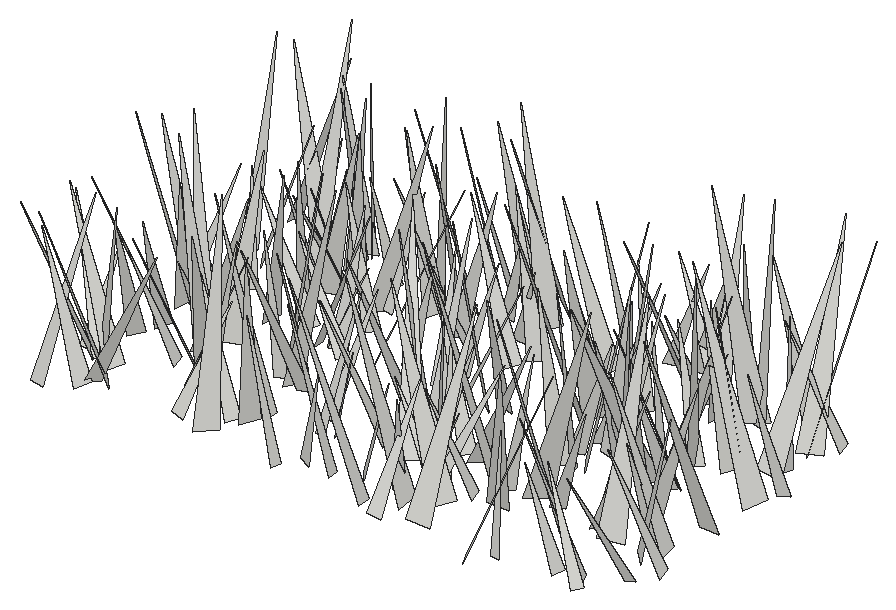
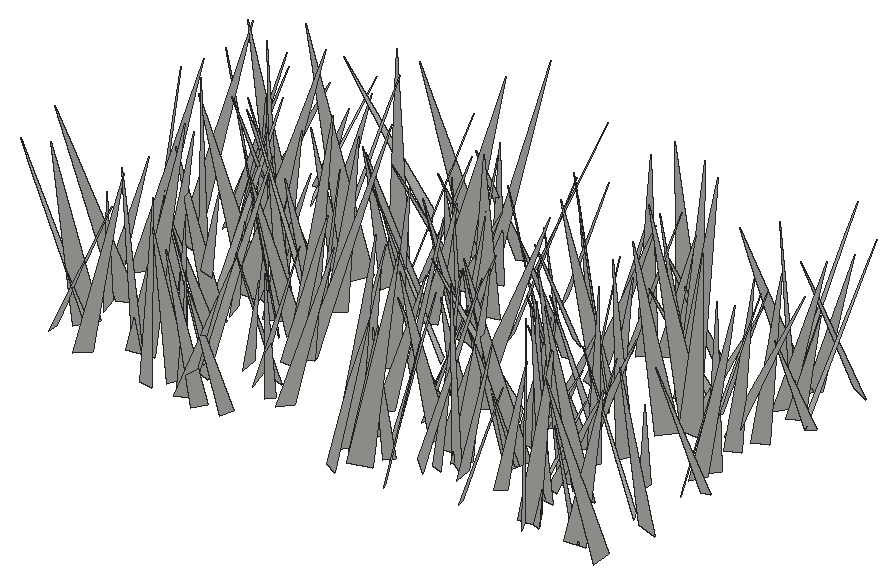
# SketchUp Ruby script. Lengths in inches.
U = 1.inch
M = Sketchup.active_model
def pt(a) = Geom::Point3d.new(a.map { |v| v * U })
def face(e, loops, mat)
  f = e.add_face(loops[0].map { |a| pt(a) })
  loops[1..].each { |l| e.add_face(l.map { |a| pt(a) }).erase! }
  f.material = f.back_material = mat if mat
  f
end
# faces: each face lists its corners as indices into pts; further lists are holes
def faces(e, pts, list, mat = nil) = list.each { |f| face(e, (f[0].is_a?(Array) ? f : [f]).map { |l| l.map { |i| pts[i] } }, mat) }
# xy, xz, yz: faces in a plane at the given z, y or x. An outline is a flat list of corners, or four numbers for a rectangle; further outlines are holes
def ring(l) = l.size == 4 ? [[l[0], l[1]], [l[2], l[1]], [l[2], l[3]], [l[0], l[3]]] : l.each_slice(2).to_a
def flat(e, list, mat, &to3) = list.each { |f| face(e, (f[0].is_a?(Array) ? f : [f]).map { |l| ring(l).map { |u, v| to3.(u, v) } }, mat) }
def xy(e, z, list, mat = nil) = flat(e, list, mat) { |x, y| [x, y, z] }
def xz(e, y, list, mat = nil) = flat(e, list, mat) { |x, z| [x, y, z] }
def yz(e, x, list, mat = nil) = flat(e, list, mat) { |y, z| [x, y, z] }
def lines(e, pts, list) = list.each { |a, b| e.add_line(pt(pts[a]), pt(pts[b])) }
# prism: a flat outline (further loops are holes) pulled along v
def prism(e, loops, v, mat = nil)
  f = face(e, loops, mat); d = Geom::Vector3d.new(v.map { |x| x * U })
  f.pushpull(f.normal.samedirection?(d) ? d.length : -d.length)
end
def box(e, o, s, mat = nil) = prism(e, [[o, [o[0] + s[0], o[1], o[2]], [o[0] + s[0], o[1] + s[1], o[2]], [o[0], o[1] + s[1], o[2]]]], [0, 0, s[2]], mat)
def at(x, y, z, deg = 0) = Geom::Transformation.translation(pt([x, y, z])) * Geom::Transformation.rotation(ORIGIN, Z_AXIS, deg.degrees)
def axes(o, x, y, z) = Geom::Transformation.new([*x, 0, *y, 0, *z, 0, *pt(o).to_a, 1])
def part(name) = M.definitions.add(name)
# library, detail: a bought-in or finely detailed component or shape, given as its bounding box
def library(name, o, s) = part(name).tap { |d| box(d.entities, o, s) }
def detail(e, o, s) = box(e.add_group.entities, o, s)
def put(e, d, t, mat = nil) = e.add_instance(d, t).tap { |i| i.material = mat if mat }
def group(e, t, mat = nil) = e.add_group.tap { |g| g.transformation = t; g.material = mat if mat }.entities
root = M.entities
c1 = part("fur_instance\#9")
p = [[0.8125,0,1.79],[0.67,-0.02,1.48],[0,-0.11,0],[0,0.11,0]]
faces(c1.entities,p,[[0,1,2,3]])
put(root,c1,axes([494.55,409.32,-21.66],[-3.60372,1.36671,1.25031],[1.68423,3.55609,0.96723],[0.77106,-1.37995,3.73084]))
put(root,c1,axes([458.37,410.72,-21.66],[-4.85913,-4.7221,0.69622],[-4.68141,4.90862,0.61965],[0.93132,0.03646,6.74725]))
put(root,c1,axes([496.72,408.43,-21.66],[-1.92431,3.57441,0.40694],[3.46774,1.72017,1.28872],[-0.95749,-0.95373,3.84949]))
put(root,c1,axes([479.86,408.75,-21.66],[-7.1325,-1.97369,0.04131],[-1.9512,7.0246,-1.27181],[-0.29997,1.23662,7.29044]))
put(root,c1,axes([457.51,409.38,-21.66],[-4.78062,2.36193,1.12593],[2.54726,4.73726,0.87783],[0.59826,-1.2963,5.25951]))
put(root,c1,axes([490.34,408.35,-21.66],[1.055,3.81063,1.04337],[3.83467,-1.24762,0.6792],[-0.95124,-0.80317,3.89521]))
put(root,c1,axes([489.08,407.03,-21.66],[5.73522,3.47371,0.17785],[3.39582,-5.66618,1.16354],[-0.75282,0.90483,6.60345]))
put(root,c1,axes([481.44,407.72,-21.66],[-0.33332,4.6985,0.41104],[4.65173,0.39553,-0.74898],[0.77866,-0.35159,4.65038]))
put(root,c1,axes([496.18,409.8,-21.66],[-4.80301,-2.64529,0.12183],[-2.62964,4.73476,-0.865],[-0.31202,0.81591,5.41463]))
put(root,c1,axes([481.99,410.3,-21.66],[-7.83608,-0.63477,1.59162],[-0.4911,7.96997,0.76075],[1.64165,-0.64574,7.82485]))
put(root,c1,axes([472.91,408.91,-21.66],[-4.76571,-0.2474,0.30777],[-0.30187,4.68534,-0.90794],[0.25457,0.92426,4.68496]))
put(root,c1,axes([498.58,411.23,-21.66],[-0.19761,-4.29399,0.26182],[-4.09062,0.10641,-1.34218],[-1.33181,0.31028,4.08362]))
put(root,c1,axes([480.77,411.1,-21.66],[0.8236,-4.35079,0.44599],[-4.32851,-0.74586,0.71716],[0.62636,0.56649,4.3696]))
put(root,c1,axes([473.95,410.375,-21.66],[-0.58036,-3.55618,1.37675],[-3.59236,0.97706,1.00942],[1.27936,1.13031,3.45894]))
put(root,c1,axes([457.67,410.2,-21.66],[5.28703,-2.12696,0.17156],[-2.11759,-5.17319,1.12251],[0.26309,1.10465,5.58719]))
put(root,c1,axes([455.2,407.84,-21.66],[2.05142,5.93925,0.09208],[5.90467,-2.04959,0.65232],[-0.64654,0.12643,6.2496]))
put(root,c1,axes([484.12,408.71,-21.66],[-1.25446,7.26591,1.58891],[7.27727,1.53186,-1.25954],[1.53602,-1.32352,7.26503]))
put(root,c1,axes([476.24,410.25,-21.66],[-5.31837,-1.43549,0.4315],[-1.49067,5.23198,-0.96754],[0.15722,1.04767,5.42306]))
put(root,c1,axes([483.2,409.68,-21.66],[3.56009,0.21869,0.65734],[0.01468,-3.46445,1.07311],[-0.69261,1.05069,3.40155]))
put(root,c1,axes([455.43,412.93,-21.66],[-4.61159,-4.4726,0.38091],[-4.39573,4.61032,0.9157],[0.90928,-0.396,6.35865]))
put(root,c1,axes([466.86,409.73,-21.66],[-5.99811,4.4385,2.51735],[4.45899,6.44808,-0.74453],[2.48087,-0.8583,7.4245]))
put(root,c1,axes([468.24,412.22,-21.66],[5.51508,-3.1001,1.56666],[-3.03836,-5.73026,-0.64316],[-1.68328,0.18611,6.29389]))
put(root,c1,axes([477.88,411.24,-21.66],[3.15545,2.01724,0.79775],[2.15051,-3.09372,-0.68323],[-0.2846,-1.01105,3.6823]))
put(root,c1,axes([464.3,410.09,-21.66],[0.4921,4.23207,0.57816],[4.10963,-0.31046,-1.22532],[1.16432,-0.69285,4.08059]))
put(root,c1,axes([483.78,411.57,-21.66],[-6.02527,4.37662,1.94606],[4.73834,5.90349,1.39383],[0.70004,-2.28907,7.31546]))
put(root,c1,axes([486.54,413.44,-21.66],[1.84605,-6.6162,0.27609],[-6.51912,-1.76548,1.28157],[1.16252,0.60597,6.74831]))
put(root,c1,axes([456.93,412.07,-21.66],[3.49606,4.56093,2.47636],[5.16488,-3.35013,-1.12142],[-0.50841,-2.67048,5.63622]))
put(root,c1,axes([467.35,411.68,-21.66],[-4.02277,2.62654,1.01722],[2.78428,3.97624,0.74391],[0.42575,-1.18612,4.74637]))
put(root,c1,axes([499.65,413.16,-21.66],[-4.7933,-0.97536,0.74224],[-0.77682,4.73507,1.20565],[0.94805,-1.05153,4.74061]))
put(root,c1,axes([484.64,413.62,-21.66],[-4.25051,-1.02119,0.70994],[-0.79222,4.17184,1.25768],[0.95876,-1.08007,4.18663]))
put(root,c1,axes([462.7,415.08,-21.66],[5.93446,-4.51627,0.11992],[-4.41947,-5.84426,-1.3935],[-0.93776,-1.03771,7.32616]))
put(root,c1,axes([457.64,412.39,-21.66],[-5.5849,2.54638,0.93821],[2.66389,5.55377,0.78405],[0.51763,-1.10771,6.08773]))
put(root,c1,axes([482.02,412.98,-21.66],[-2.52559,2.65872,0.46687],[2.62617,2.27215,1.26725],[-0.62447,-1.19747,3.44114]))
put(root,c1,axes([491.17,413.7,-21.66],[-5.74367,-4.09689,1.01684],[-4.21686,5.6466,-1.0688],[0.19121,1.46278,6.97366]))
put(root,c1,axes([464.03,413.46,-21.66],[-1.49797,-4.88201,2.75569],[-5.27998,2.18724,1.00478],[1.88406,2.24805,5.00683]))
put(root,c1,axes([497.22,413.81,-21.66],[4.01593,3.70117,1.52807],[3.99587,-3.8439,-1.19115],[-0.25835,-1.92018,5.32987]))
put(root,c1,axes([482.36,412.28,-21.66],[1.65691,4.63189,0.02775],[4.518,-1.60961,-1.09423],[1.0212,-0.39403,4.79608]))
put(root,c1,axes([476.14,415.5,-21.66],[-5.06216,-2.56794,0.53616],[-2.44101,5.03776,1.08155],[0.96086,-0.73072,5.57226]))
put(root,c1,axes([473.18,414.41,-21.66],[3.34183,1.38887,0.77255],[1.56239,-3.2005,-1.00466],[-0.29109,-1.23347,3.4767]))
put(root,c1,axes([456.21,412.79,-21.66],[-3.43494,4.07646,0.13435],[4.04677,3.38429,0.77755],[-0.50915,-0.60283,5.27368]))
put(root,c1,axes([460.22,415.27,-21.66],[-4.26767,-0.91045,0.71231],[-0.70932,4.21373,1.13607],[0.91278,-0.98229,4.21323]))
put(root,c1,axes([468.82,413.53,-21.66],[-7.05105,-1.29004,0.36767],[-1.33665,6.92247,-1.34515],[0.11284,1.38992,7.04075]))
put(root,c1,axes([496.81,415.76,-21.66],[3.89618,-1.88557,1.1779],[-1.51971,-3.99347,-1.36592],[-1.62275,-0.78732,4.1073]))
put(root,c1,axes([454.74,413.15,-21.66],[-0.81178,3.59213,0.55552],[3.51446,0.92094,-0.81938],[0.92765,-0.34562,3.5904]))
put(root,c1,axes([498.1875,415.4,-21.66],[-6.30832,-1.1114,1.05664],[-1.00602,6.37534,0.69964],[1.15742,-0.51611,6.36715]))
put(root,c1,axes([456.05,416.43,-21.66],[3.84252,-3.67557,0.42443],[-3.56655,-3.84235,-0.9854],[-0.98471,-0.42605,5.2253]))
put(root,c1,axes([482.69,413.06,-21.66],[-4.63028,1.37895,0.71291],[1.15549,4.55932,-1.31404],[1.03661,1.07721,4.64912]))
put(root,c1,axes([461.4,415.51,-21.66],[-3.04212,-3.44962,0.11938],[-3.35963,2.92271,-1.15727],[-0.79185,0.85236,4.45141]))
put(root,c1,axes([489.52,415.54,-21.66],[3.13596,-3.23192,0.2957],[-3.22644,-3.06024,0.76944],[0.35051,0.74607,4.43707]))
put(root,c1,axes([462.7,415.23,-21.66],[1.59006,-7.38899,3.46765],[-7.94346,-2.21328,-1.07372],[-1.87702,3.10714,7.48148]))
put(root,c1,axes([487.81,415.73,-21.66],[6.25642,-5.32962,1.03257],[-5.42827,-6.12142,1.29455],[0.06986,1.65444,8.11614]))
put(root,c1,axes([462.29,413.48,-21.66],[4.05537,2.07279,0.17475],[1.9711,-3.95155,1.12829],[-0.66463,0.92835,4.41242]))
put(root,c1,axes([472.55,413.58,-21.66],[1.79845,4.31058,0.12569],[4.2592,-1.79684,0.67963],[-0.67534,0.14702,4.621]))
put(root,c1,axes([468.5,417.22,-21.66],[-0.3519,-5.66898,0.64957],[-5.59847,0.21723,-1.13712],[-1.1029,0.70611,5.5649]))
put(root,c1,axes([484.61,415.62,-21.66],[-7.32124,-3.15954,0.71739],[-3.23761,7.2018,-1.32279],[0.12329,1.49974,7.86343]))
put(root,c1,axes([485.79,415.33,-21.66],[4.38322,-1.64948,1.59394],[-1.93146,-4.50849,0.64578],[-1.2373,1.19448,4.63858]))
put(root,c1,axes([494.61,414.32,-21.66],[-2.78975,7.45432,2.27613],[7.61508,3.12201,-0.8911],[1.66081,-1.79348,7.90921]))
put(root,c1,axes([492.91,415.11,-21.66],[5.00649,-0.69371,1.01239],[-0.92226,-4.93206,1.18126],[-0.80969,1.32843,4.91435]))
put(root,c1,axes([456.72,418.28,-21.66],[4.17409,-3.35782,0.27535],[-3.2273,-4.11088,-1.20788],[-0.96712,-0.77425,5.2191]))
put(root,c1,axes([457.68,417.55,-21.66],[-3.27123,-4.88451,0.3113],[-4.82797,3.15879,-1.17003],[-0.80376,0.90546,5.76111]))
put(root,c1,axes([460.55,417.32,-21.66],[5.42547,-4.53511,0.52895],[-4.56014,-5.3411,0.98008],[0.2284,1.09004,7.00303]))
put(root,c1,axes([471.8,415.45,-21.66],[0.88242,4.55252,0.64978],[4.54635,-0.76413,-0.82042],[0.6916,-0.78549,4.5641]))
put(root,c1,axes([480.07,415.68,-21.66],[-4.86729,-1.78674,2.25978],[-2.35287,5.02555,-1.09424],[1.66225,1.88173,5.06809]))
put(root,c1,axes([479.28,416.67,-21.66],[0.33455,3.97904,1.71347],[4.11253,0.24873,-1.38056],[1.36232,-1.72801,3.74683]))
put(root,c1,axes([482.08,416.86,-21.66],[4.93305,-2.19664,0.15391],[-2.18894,-4.85066,0.92924],[0.23965,0.9109,5.31946]))
put(root,c1,axes([478.96,416.41,-21.66],[-6.73527,-1.87686,1.53677],[-2.12146,6.75676,-1.04577],[1.17629,1.43931,6.91323]))
put(root,c1,axes([498.45,419.07,-21.66],[-0.93689,-7.58778,0.99671],[-7.63501,0.85799,-0.64504],[-0.52389,1.06539,7.61814]))
put(root,c1,axes([478.85,414.61,-21.66],[-3.36629,7.35026,0.38103],[7.33966,3.3212,0.77612],[-0.54849,-0.66835,8.0471]))
put(root,c1,axes([492.17,418.33,-21.66],[7.07527,1.73735,2.55738],[2.12787,-7.36989,-0.88027],[-2.24293,-1.5114,7.23207]))
put(root,c1,axes([481.05,417.37,-21.66],[-3.33055,3.67395,0.98734],[3.8043,3.21801,0.85849],[0.0046,-1.30837,4.884]))
put(root,c1,axes([467.34,419.05,-21.66],[3.26712,2.26093,2.86418],[3.20778,-3.61207,-0.80776],[-1.73938,-2.41465,3.89016]))
put(root,c1,axes([478.22,417.79,-21.66],[-2.47066,2.78913,0.64805],[2.82871,2.24449,1.12431],[-0.44456,-1.21919,3.55237]))
put(root,c1,axes([466.3,417.65,-21.66],[-0.19493,4.51759,1.73565],[4.75586,-0.14282,0.90585],[-0.89608,-1.74071,4.43013]))
put(root,c1,axes([494.83,418.04,-21.66],[4.67154,-2.82363,0.84685],[-2.94301,-4.55853,1.0353],[-0.16964,1.32674,5.35951]))
put(root,c1,axes([467.43,417.39,-21.66],[6.54484,-1.1484,2.12677],[-1.53141,-6.71985,1.08414],[-1.86996,1.48383,6.55579]))
put(root,c1,axes([491.85,421.64,-21.66],[1.8393,-7.94223,0.20343],[-7.82957,-1.84746,-1.33722],[-1.34842,-0.10629,8.04201]))
put(root,c1,axes([465.96,418.75,-21.66],[6.04593,4.4435,2.18806],[4.86244,-5.98205,-1.28733],[-0.94282,-2.35709,7.39194]))
put(root,c1,axes([474.54,419.79,-21.66],[-1.00098,-5.50903,0.83943],[-5.47181,0.81017,-1.20786],[-1.05515,1.02481,5.46739]))
put(root,c1,axes([492.6,416.15,-21.66],[3.19327,6.60837,0.52108],[6.51338,-3.23542,1.11669],[-1.23207,0.02336,7.254]))
put(root,c1,axes([460.02,418.17,-21.66],[-1.69454,7.12423,1.83382],[7.32335,1.45532,1.11334],[-0.69716,-2.02889,7.23786]))
put(root,c1,axes([491.04,421.41,-21.66],[0.94954,-6.1364,0.24208],[-6.03443,-0.88683,1.18943],[1.14,0.41683,6.09444]))
put(root,c1,axes([486.33,419.76,-21.66],[-4.53938,3.59005,2.40826],[4.08452,4.7056,0.68422],[1.41595,-2.06469,5.74685]))
put(root,c1,axes([461.17,419.04,-21.66],[-3.27295,5.40819,2.7555],[5.57889,3.91368,-1.05481],[2.39109,-1.7286,6.23283]))
put(root,c1,axes([456.03,421.01,-21.66],[5.00192,-1.81934,1.03799],[-1.65,-5.07776,-0.94895],[-1.29032,-0.55947,5.23724]))
put(root,c1,axes([493.34,421.6,-21.66],[2.17041,-4.52553,0.56409],[-4.42394,-2.24099,-0.95709],[-1.10786,0.0828,4.92697]))
put(root,c1,axes([457.46,420.44,-21.66],[-5.88104,-3.53705,0.94417],[-3.64814,5.81133,-0.9531],[0.30541,1.30636,6.79625]))
put(root,c1,axes([493.27,422.5,-21.66],[-4.06699,-5.2197,0.56162],[-5.13541,4.10303,0.94539],[1.09007,-0.14467,6.54919]))
put(root,c1,axes([487.39,419.78,-21.66],[-5.21816,-1.76906,1.50642],[-2.07355,5.2165,-1.05669],[1.04846,1.51216,5.4076]))
put(root,c1,axes([477.78,417.8125,-21.66],[1.53889,6.65129,0.3221],[6.53467,-1.57198,1.24039],[-1.28121,-0.02868,6.71336]))
put(root,c1,axes([488.67,422.94,-21.66],[4.29462,-4.11505,0.26594],[-3.98176,-4.23808,-1.27765],[-1.07236,-0.74374,5.80905]))
put(root,c1,axes([477.53,420.49,-21.66],[5.0651,3.0377,0.15182],[3.00547,-4.95362,-1.15532],[0.46672,-1.0677,5.79207]))
put(root,c1,axes([490.27,421.64,-21.66],[-1.57238,-4.56901,1.11948],[-4.65933,1.35009,-1.0341],[-0.64787,1.37945,4.72005]))
put(root,c1,axes([479.28,423.125,-21.66],[-0.0268,-5.65268,0.22398],[-5.53849,0.07185,1.15049],[1.15241,0.21383,5.53443]))
put(root,c1,axes([486.15,421.55,-21.66],[3.07396,-3.53335,0.83024],[-3.61315,-2.87553,1.13994],[0.34489,1.36741,4.5425]))
put(root,c1,axes([456.26,422.18,-21.66],[-6.02827,1.48886,1.73676],[1.72693,6.17226,0.7029],[1.50026,-1.12234,6.1695]))
put(root,c1,axes([461.34,422.98,-21.66],[5.97247,-1.71505,1.0533],[-1.60325,-6.04797,-0.7569],[-1.21673,-0.44932,6.16757]))
put(root,c1,axes([467.66,421.95,-21.66],[-3.1989,2.68909,0.37978],[2.66785,3.00183,1.21655],[-0.50792,-1.16886,3.99802]))
put(root,c1,axes([487.98,422.43,-21.66],[-0.07815,-6.05054,2.52953],[-6.4447,0.53908,1.09033],[1.2138,2.47266,5.952]))
put(root,c1,axes([487.625,420.57,-21.66],[6.38887,5.18246,1.59043],[5.07791,-6.58181,1.04866],[-1.89794,-0.16426,8.1594]))
put(root,c1,axes([497.56,423.78,-21.66],[4.54557,4.08977,3.87164],[5.12111,-5.0718,-0.65499],[-2.34307,-3.15097,6.07942]))
put(root,c1,axes([478.53,422.4375,-21.66],[2.96491,4.33641,3.25393],[4.46173,-4.05854,1.34327],[-3.07985,-1.70497,5.07846]))
put(root,c1,axes([484.5,424.36,-21.66],[-4.58981,-6.81856,1.14154],[-6.9132,4.53833,-0.68805],[0.05895,1.33156,8.19058]))
put(root,c1,axes([465.78,422.92,-21.66],[3.19259,1.80159,0.09548],[1.75198,-3.04965,-1.03811],[0.43061,-0.9494,3.51578]))
put(root,c1,axes([498.67,423.29,-21.66],[-7.81883,2.51294,1.68172],[2.76611,7.82758,1.16397],[1.22135,-1.64052,8.12983]))
put(root,c1,axes([471.63,423.47,-21.66],[1.56073,-4.1385,0.9971],[-4.17951,-1.28812,1.1957],[0.80812,1.33073,4.25833]))
put(root,c1,axes([465.54,422.23,-21.66],[4.89085,0.64493,0.58721],[0.56841,-4.89366,0.64042],[-0.66156,0.56328,4.89144]))
put(root,c1,axes([466.84,422.5625,-21.66],[-2.42701,4.03219,1.90827],[4.11447,2.86278,-0.81615],[1.72373,-1.15601,4.63496]))
put(root,c1,axes([484.32,425.72,-21.66],[5.05065,-5.78899,0.88016],[-5.66798,-5.12516,-1.18448],[-1.47008,-0.1285,7.59069]))
put(root,c1,axes([486.57,423.39,-21.66],[4.08139,-3.20586,0.61223],[-3.2526,-3.91407,1.18774],[0.27008,1.30866,5.05219]))
put(root,c1,axes([455.82,424.36,-21.66],[-3.08221,-2.2445,0.63722],[-2.14243,3.14072,0.69983],[0.92405,-0.20483,3.74807]))
put(root,c1,axes([463.95,423.6,-21.66],[-4.51711,1.79985,0.33219],[1.82954,4.41557,0.95372],[-0.05124,-1.00862,4.76803]))
put(root,c1,axes([464.62,421.78,-21.66],[4.77639,3.07128,1.21309],[2.81816,-4.90311,1.31748],[-1.72115,0.49496,5.52367]))
put(root,c1,axes([492.72,424.6,-21.66],[7.08469,1.17747,2.52447],[1.61288,-7.35894,-1.094],[-2.27113,-1.55299,7.09806]))
put(root,c1,axes([475.82,423.58,-21.66],[-4.15206,-1.52587,0.16301],[-1.50616,3.96212,-1.27574],[-0.29385,1.25209,4.2356]))
put(root,c1,axes([462.26,424.89,-21.66],[5.48977,-0.87036,1.92832],[-0.64898,-5.79667,-0.76876],[-2.01365,-0.50463,5.50492]))
put(root,c1,axes([454.75,423.33,-21.66],[1.35315,4.35582,0.79538],[4.34518,-1.14634,-1.11449],[0.85157,-1.07217,4.42291]))
put(root,c1,axes([474.34,422.88,-21.66],[-3.56654,2.39752,0.7344],[2.22273,3.6139,-1.00345],[1.16058,0.44646,4.17868]))
put(root,c1,axes([499.32,425.23,-21.66],[0.38107,-4.3176,1.24457],[-4.35966,-0.65774,-0.94692],[-1.08815,1.12319,4.22969]))
put(root,c1,axes([491.2,423.59,-21.66],[-4.4304,-0.23548,0.66281],[-0.42328,4.26855,-1.31284],[0.56178,1.35914,4.23796]))
put(root,c1,axes([469.55,422.78,-21.66],[5.6659,3.07924,0.02777],[3.03508,-5.59401,1.03936],[-0.52039,0.90013,6.36426]))
put(root,c1,axes([491.08,425.44,-21.66],[4.31446,-3.71791,0.40504],[-3.72385,-4.21342,0.9907],[0.3462,1.01276,5.60856]))
put(root,c1,axes([487.67,423.76,-21.66],[-4.49953,-3.59508,3.80394],[-4.60675,5.10137,-0.62788],[2.48443,2.94818,5.72505]))
put(root,c1,axes([494.8125,425.6875,-21.66],[4.62611,-3.05223,2.53258],[-2.97331,-5.24406,-0.88892],[-2.62479,0.5609,5.47054]))
put(root,c1,axes([492.79,424.86,-21.66],[1.4221,-3.78822,2.5832],[-4.25079,-2.10312,-0.74405],[-1.71882,2.06693,3.97736]))
put(root,c1,axes([466.5,425.57,-21.66],[-2.71564,-2.49022,0.0198],[-2.39499,2.6036,-1.03032],[-0.68234,0.77224,3.53756]))
put(root,c1,axes([473.71,427.05,-21.66],[-3.49973,-1.74713,0.54329],[-1.50598,3.41664,1.28623],[1.03907,-0.93268,3.69408]))
put(root,c1,axes([474.87,424.56,-21.66],[3.51726,-1.23078,1.44078],[-1.67757,-3.4351,1.16087],[-0.88116,1.62697,3.54095]))
put(root,c1,axes([467.04,425.54,-21.66],[1.69917,-3.99461,2.49122],[-4.30676,-2.38859,-0.89256],[-1.90128,1.84064,4.24822]))
put(root,c1,axes([484.5,426.66,-21.66],[0.91416,-4.94391,1.27953],[-4.9749,-1.15567,-0.91103],[-1.1532,1.06645,4.94449]))
put(root,c1,axes([458.07,425.1,-21.66],[-3.61922,1.27993,0.57976],[1.16278,3.62754,-0.74965],[0.78884,0.52519,3.76496]))
put(root,c1,axes([461.9,427.53,-21.66],[4.17452,-5.37379,1.20818],[-5.50555,-4.02647,1.11376],[0.16212,1.6352,6.71296]))
put(root,c1,axes([489.99,427.18,-21.66],[3.34433,-2.45993,0.06359],[-2.39384,-3.22746,1.0454],[0.56992,0.87868,4.01783]))
put(root,c1,axes([460.62,428.27,-21.66],[-3.9819,-2.09854,0.99873],[-1.89028,4.07705,1.03024],[1.35209,-0.4803,4.38155]))
put(root,c1,axes([470.4375,429.03,-21.66],[1.77342,-4.13167,0.71101],[-4.001,-1.89854,-1.053],[-1.2523,0.21471,4.37115]))
put(root,c1,axes([476.4,427.47,-21.66],[-4.85696,2.92878,0.85344],[3.03677,4.79447,0.82904],[0.29007,-1.15391,5.61075]))
put(root,c1,axes([462.3,428.8125,-21.66],[-0.70477,-3.63934,0.22038],[-3.52996,0.62491,-0.96896],[-0.91253,0.39339,3.57807]))
put(root,c1,axes([463.36,428.0625,-21.66],[-3.08913,-1.9262,0.20442],[-1.91689,2.98464,-0.84391],[-0.27849,0.82245,3.5413]))
put(root,c1,axes([465.73,427.72,-21.66],[6.31096,-2.97385,1.65761],[-3.28181,-6.24286,1.29466],[-0.9062,1.89806,6.85536]))
put(root,c1,axes([487.78,430.95,-21.66],[-3.38776,-6.42257,0.32475],[-6.36234,3.40084,0.88702],[0.93573,-0.12917,7.20691]))
put(root,c1,axes([456.41,428.17,-21.66],[4.70564,3.18962,0.73071],[3.27223,-4.59158,-1.02983],[-0.01227,-1.26267,5.59072]))
put(root,c1,axes([471.5,428.24,-21.66],[4.65487,-3.05281,1.35089],[-3.29302,-4.57961,0.99778],[-0.54826,1.58741,5.47649]))
put(root,c1,axes([466.07,428.04,-21.66],[-0.49271,4.25835,1.65602],[4.30491,0.99075,-1.26683],[1.53091,-1.41548,4.0953]))
put(root,c1,axes([490.07,430.13,-21.66],[3.94789,-1.4658,0.35037],[-1.34081,-3.86465,-1.06014],[-0.68816,-0.87925,4.0756]))
put(root,c1,axes([468.7,429.6,-21.66],[-5.74569,2.33772,2.68731],[2.89131,6.03979,0.92776],[2.08013,-1.9379,6.13328]))
put(root,c1,axes([497.58,427.82,-21.66],[-4.70779,-0.34884,1.44292],[-0.70643,4.74641,-1.15738],[1.30563,1.3103,4.57662]))
put(root,c1,axes([462.11,430.21,-21.66],[1.6892,-5.96403,1.00433],[-6.01842,-1.55459,0.89085],[0.59746,1.20222,6.13428]))
put(root,c1,axes([496.96,426.76,-21.66],[-0.59068,7.87895,1.19707],[7.83923,0.79048,-1.33468],[1.43434,-1.07565,7.78752]))
put(root,c1,axes([483.6,428.76,-21.66],[2.51167,3.62255,0.80621],[3.69421,-2.34748,-0.96099],[0.35452,-1.20325,4.30208]))
put(root,c1,axes([477.14,428.93,-21.66],[1.60632,-4.77246,2.92285],[-5.28453,-2.29441,-0.84211],[-1.84207,2.42054,4.96463]))
put(root,c1,axes([469.46,431.06,-21.66],[-2.94569,-5.43055,1.36405],[-5.282,3.20651,1.35919],[1.85796,0.50597,6.02666]))
put(root,c1,axes([474.76,430.2,-21.66],[1.46313,-3.34357,0.17988],[-3.25058,-1.37123,0.95187],[0.80348,0.54115,3.52337]))
put(root,c1,axes([488.31,429.9,-21.66],[4.57096,2.53062,0.74602],[2.63797,-4.36083,-1.37058],[0.04077,-1.55993,5.04174]))
put(root,c1,axes([482.78,430.6,-21.66],[3.65052,-1.24636,0.3015],[-1.17659,-3.61738,-0.70767],[-0.50984,-0.576,3.79195]))
put(root,c1,axes([486.3125,428.28,-21.66],[-4.58917,0.765,0.19448],[0.68534,4.43094,-1.25723],[0.3916,1.21042,4.47941]))
put(root,c1,axes([464.78,430.71,-21.66],[3.15907,-2.58161,1.45094],[-2.40771,-3.47422,-0.93937],[-1.72421,0.12146,3.97014]))
put(root,c1,axes([461.76,430.13,-21.66],[2.13967,5.72529,2.72362],[6.33838,-1.99885,-0.77766],[-0.14822,-2.82858,6.06237]))
put(root,c1,axes([484.8,429.26,-21.66],[-6.17227,-0.98801,0.5453],[-1.07692,6.06305,-1.2042],[0.3373,1.27815,6.13375]))
put(root,c1,axes([488.39,431.22,-21.66],[0.67909,-3.62862,0.46379],[-3.53581,-0.77205,-0.86319],[-0.93808,0.2832,3.58928]))
put(root,c1,axes([481.48,430.75,-21.66],[-5.50696,2.25656,1.40845],[2.52369,5.45565,1.12666],[0.84072,-1.59571,5.84374]))
put(root,c1,axes([492.36,431.25,-21.66],[2.49125,-7.31611,3.2771],[-7.62751,-3.2193,-1.38865],[-2.46697,2.5655,7.60286]))
put(root,c1,axes([470.43,431.44,-21.66],[-4.6315,-5.30606,1.24554],[-5.44783,4.55599,-0.84886],[0.16366,1.49838,6.99175]))
put(root,c1,axes([460.3,428.22,-21.66],[0.64716,8.27924,1.09317],[8.31403,-0.74193,0.69715],[-0.78591,-1.0312,8.27518]))
put(root,c1,axes([461.21,431.46,-21.66],[2.3019,2.88607,2.09295],[3.52279,-2.224,-0.8077],[-0.54756,-2.17555,3.60219]))
put(root,c1,axes([454.7,429.15,-21.66],[1.29784,6.7007,1.25957],[6.74597,-1.44798,0.75208],[-0.98888,-1.08363,6.78367]))
put(root,c1,axes([468.62,430.23,-21.66],[2.86323,5.98862,2.41998],[6.20716,-3.28322,0.78076],[-1.78634,-1.80966,6.59182]))
put(root,c1,axes([498.45,432.1,-21.66],[-4.68733,-0.90911,0.30449],[-0.85582,4.65242,0.7161],[0.43216,-0.64711,4.72067]))
put(root,c1,axes([472.43,432.01,-21.66],[0.98375,-3.96673,0.69714],[-3.91068,-0.76919,1.14174],[0.96305,0.9285,3.92417]))
put(root,c1,axes([467.69,430.75,-21.66],[-5.58164,-0.15602,0.84627],[-0.25003,5.60842,-0.61509],[0.82341,0.64537,5.54984]))
put(root,c1,axes([460.52,432.87,-21.66],[-2.8459,-6.01928,1.64103],[-5.98512,3.14324,1.14988],[1.76154,0.95508,6.5581]))
put(root,c1,axes([472.79,431.54,-21.66],[-4.95008,-4.07189,1.35786],[-4.2827,4.82407,-1.14641],[0.2873,1.75371,6.30629]))
put(root,c1,axes([474.5,432.53,-21.66],[-2.85824,2.70123,1.97363],[3.21945,2.92659,0.65696],[0.90938,-1.87078,3.87745]))
put(root,c1,axes([487.84,432.97,-21.66],[3.54062,0.10617,1.20258],[0.38468,-3.63127,-0.812],[-1.14433,-0.89222,3.44788]))
put(root,c1,axes([465.68,433.51,-21.66],[-3.61169,-1.5954,0.61372],[-1.41522,3.59542,1.01805],[0.9587,-0.70282,3.81487]))
put(root,c1,axes([497.0625,430.38,-21.66],[6.03648,4.13261,1.07509],[4.02235,-6.12795,0.97074],[-1.43354,0.20766,7.25088]))
put(root,c1,axes([495.21,433.24,-21.66],[4.87258,-2.82126,2.84071],[-2.53321,-5.63755,-1.25383],[-3.10033,0.17232,5.48903]))
put(root,c1,axes([475.28,432.55,-21.66],[-6.5147,3.53544,2.59254],[3.94464,6.75335,0.70282],[1.91322,-1.88542,7.3788]))
put(root,c1,axes([492.85,430.93,-21.66],[2.9733,6.47594,2.08154],[6.51847,-3.36189,1.14821],[-1.94427,-1.36785,7.03277]))
put(root,c1,axes([460.88,432.875,-21.66],[1.22573,-5.85041,2.29876],[-6.17569,-1.55733,-0.67049],[-1.1715,2.08841,5.93971]))
put(root,c1,axes([473.35,433.66,-21.66],[3.66547,-5.8791,2.24711],[-5.89364,-4.11869,-1.16204],[-2.20868,1.23351,6.83002]))
put(root,c1,axes([460.84,433.45,-21.66],[5.57047,2.74276,2.66238],[3.42235,-5.67452,-1.31471],[-1.7025,-2.43273,6.06831]))
put(root,c1,axes([497.28,430.3,-21.66],[-5.06165,5.7028,1.49455],[5.55918,5.27278,-1.292],[1.96243,-0.22764,7.51486]))
put(root,c1,axes([474.52,435.06,-21.66],[-3.9391,-6.11846,0.96009],[-6.01065,4.05101,1.1555],[1.49311,0.1661,7.18449]))
put(root,c1,axes([457.06,433.09,-21.66],[1.7878,3.1828,1.34143],[3.44443,-1.53093,-0.95817],[0.2561,-1.62848,3.52255]))
put(root,c1,axes([489.68,434.04,-21.66],[-1.49561,-5.63035,1.67127],[-5.71638,1.79132,0.91926],[1.34798,1.34949,5.75262]))
put(root,c1,axes([470.625,434.6875,-21.66],[-3.85431,-2.63258,1.04926],[-2.43046,3.98156,1.06172],[1.4575,-0.32233,4.54521]))
put(root,c1,axes([485.56,434.05,-21.66],[2.4486,-4.30122,0.69777],[-4.269,-2.2075,1.37318],[0.8735,1.26866,4.75506]))
put(root,c1,axes([457.02,433.21,-21.66],[-2.59565,5.50063,1.7013],[5.74289,2.3395,1.19781],[-0.41302,-2.03926,5.96319]))
put(root,c1,axes([487.13,433.81,-21.66],[-3.1283,2.85302,0.75954],[2.94685,2.94951,1.058],[-0.18092,-1.28978,4.09959]))
put(root,c1,axes([483.6875,433.7,-21.66],[3.11489,-2.67244,0.85057],[-2.80172,-2.90834,1.1224],[0.12545,1.40269,3.94774]))
put(root,c1,axes([488.51,432.38,-21.66],[-5.11212,3.73872,1.49873],[3.53116,5.32488,-1.23875],[1.93782,0.15985,6.21106]))
put(root,c1,axes([454.67,433.61,-21.66],[6.22243,-0.20354,0.93497],[-0.30289,-6.25415,0.65425],[-0.90767,0.69164,6.19128]))
